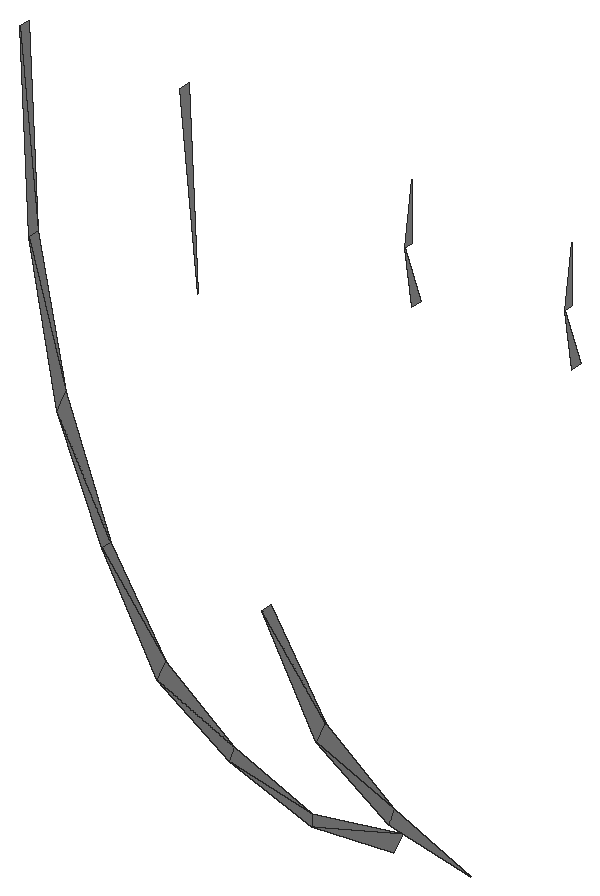
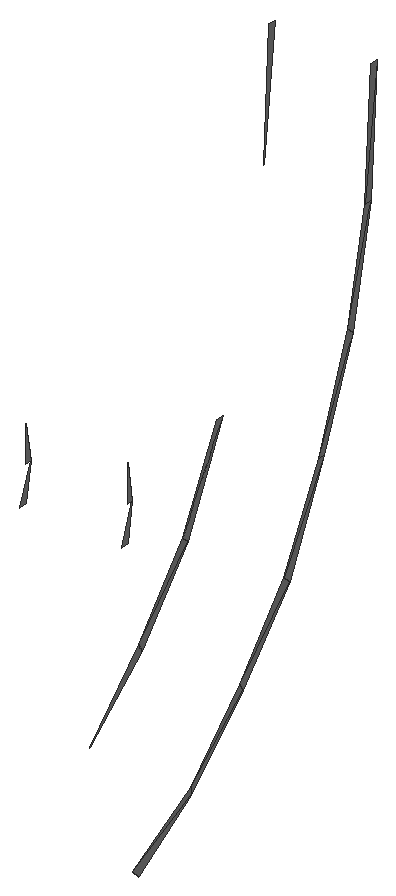
# SketchUp Ruby script. Lengths in inches.
U = 1.inch
M = Sketchup.active_model
def pt(a) = Geom::Point3d.new(a.map { |v| v * U })
def face(e, loops, mat)
  f = e.add_face(loops[0].map { |a| pt(a) })
  loops[1..].each { |l| e.add_face(l.map { |a| pt(a) }).erase! }
  f.material = f.back_material = mat if mat
  f
end
# faces: each face lists its corners as indices into pts; further lists are holes
def faces(e, pts, list, mat = nil) = list.each { |f| face(e, (f[0].is_a?(Array) ? f : [f]).map { |l| l.map { |i| pts[i] } }, mat) }
# xy, xz, yz: faces in a plane at the given z, y or x. An outline is a flat list of corners, or four numbers for a rectangle; further outlines are holes
def ring(l) = l.size == 4 ? [[l[0], l[1]], [l[2], l[1]], [l[2], l[3]], [l[0], l[3]]] : l.each_slice(2).to_a
def flat(e, list, mat, &to3) = list.each { |f| face(e, (f[0].is_a?(Array) ? f : [f]).map { |l| ring(l).map { |u, v| to3.(u, v) } }, mat) }
def xy(e, z, list, mat = nil) = flat(e, list, mat) { |x, y| [x, y, z] }
def xz(e, y, list, mat = nil) = flat(e, list, mat) { |x, z| [x, y, z] }
def yz(e, x, list, mat = nil) = flat(e, list, mat) { |y, z| [x, y, z] }
def lines(e, pts, list) = list.each { |a, b| e.add_line(pt(pts[a]), pt(pts[b])) }
# prism: a flat outline (further loops are holes) pulled along v
def prism(e, loops, v, mat = nil)
  f = face(e, loops, mat); d = Geom::Vector3d.new(v.map { |x| x * U })
  f.pushpull(f.normal.samedirection?(d) ? d.length : -d.length)
end
def box(e, o, s, mat = nil) = prism(e, [[o, [o[0] + s[0], o[1], o[2]], [o[0] + s[0], o[1] + s[1], o[2]], [o[0], o[1] + s[1], o[2]]]], [0, 0, s[2]], mat)
def at(x, y, z, deg = 0) = Geom::Transformation.translation(pt([x, y, z])) * Geom::Transformation.rotation(ORIGIN, Z_AXIS, deg.degrees)
def axes(o, x, y, z) = Geom::Transformation.new([*x, 0, *y, 0, *z, 0, *pt(o).to_a, 1])
def part(name) = M.definitions.add(name)
# library, detail: a bought-in or finely detailed component or shape, given as its bounding box
def library(name, o, s) = part(name).tap { |d| box(d.entities, o, s) }
def detail(e, o, s) = box(e.add_group.entities, o, s)
def put(e, d, t, mat = nil) = e.add_instance(d, t).tap { |i| i.material = mat if mat }
def group(e, t, mat = nil) = e.add_group.tap { |g| g.transformation = t; g.material = mat if mat }.entities
root = M.entities
M.materials.add("Material \#1").color = [140, 140, 140]
yz(root,155.64,[[443.8,49.93,443.81,49.94,443.71,49.99],[443.81,49.94,443.71,50,443.71,49.99],[443.71,49.99,443.71,50,443.62,50.08],[443.71,50,443.625,50.09,443.62,50.08],[443.62,50.08,443.625,50.09,443.54,50.18],
  [443.625,50.09,443.55,50.19,443.54,50.18],[443.54,50.18,443.55,50.19,443.48,50.31],[443.55,50.19,443.49,50.31,443.48,50.31],[443.48,50.31,443.49,50.31,443.43,50.44],[443.49,50.31,443.44,50.45,443.43,50.44],
  [443.82,50.35,443.83,50.35,443.8125,50.4],[443.8125,50.4,443.82,50.4,443.82,50.45],[443.43,50.44,443.44,50.45,443.4,50.59],[443.44,50.45,443.41,50.59,443.4,50.59],[443.4,50.59,443.41,50.59,443.39,50.76],
  [443.41,50.59,443.4,50.76,443.39,50.76]],"Material \#1")
yz(root,155.78,[[443.71,50,443.62,50.08,443.625,50.09],[443.62,50.08,443.54,50.18,443.625,50.09],[443.625,50.09,443.54,50.18,443.55,50.19],[443.54,50.18,443.48,50.31,443.55,50.19],[443.55,50.19,443.48,50.31,443.49,50.31],
  [443.82,50.35,443.8125,50.4,443.83,50.35],[443.8125,50.4,443.82,50.45,443.82,50.4],[443.41,50.59,443.39,50.76,443.4,50.76]],"Material \#1")
